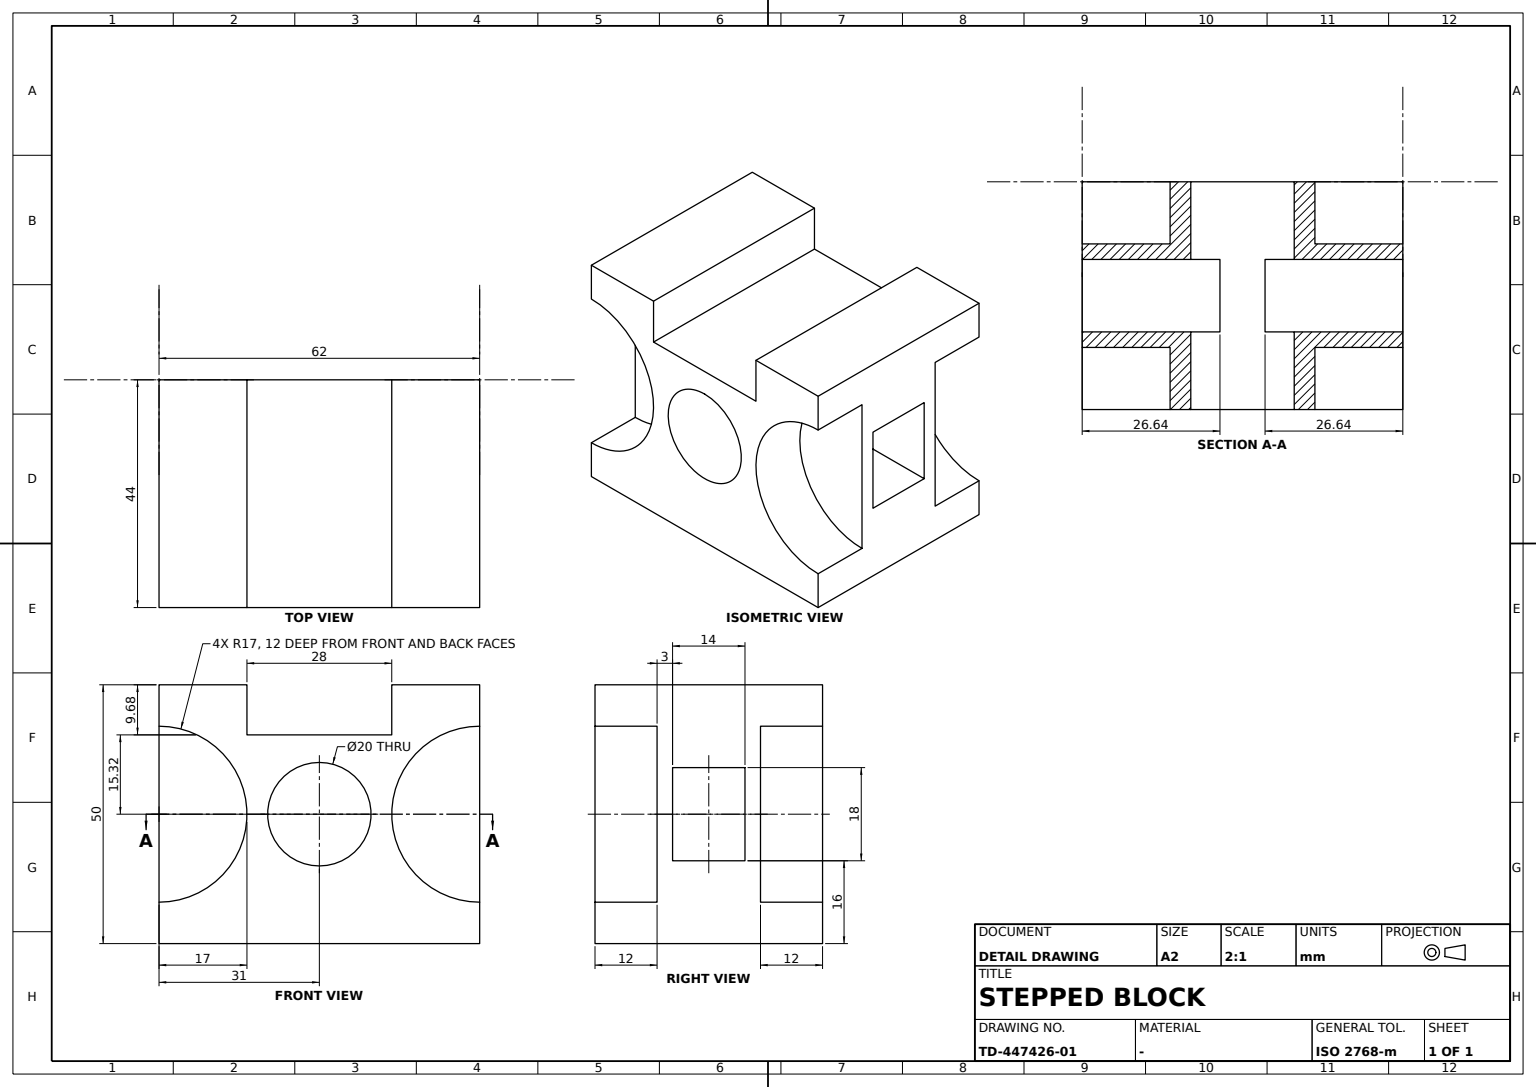
ISO-10303-21;
HEADER;
FILE_DESCRIPTION((''),'2;1');
FILE_NAME('','',(''),(''),'','','');
FILE_SCHEMA(('AUTOMOTIVE_DESIGN'));
ENDSEC;
DATA;
#1=APPLICATION_CONTEXT('');
#2=PRODUCT_CONTEXT('',#1,'mechanical');
#3=PRODUCT('','','',(#2));
#4=PRODUCT_DEFINITION_FORMATION('','',#3);
#5=PRODUCT_DEFINITION_CONTEXT('',#1,'design');
#6=PRODUCT_DEFINITION('','',#4,#5);
#7=PRODUCT_DEFINITION_SHAPE('','',#6);
#8=(LENGTH_UNIT()NAMED_UNIT(*)SI_UNIT(.MILLI.,.METRE.));
#9=(NAMED_UNIT(*)PLANE_ANGLE_UNIT()SI_UNIT($,.RADIAN.));
#10=(NAMED_UNIT(*)SI_UNIT($,.STERADIAN.)SOLID_ANGLE_UNIT());
#11=UNCERTAINTY_MEASURE_WITH_UNIT(LENGTH_MEASURE(0.005),#8,'distance_accuracy_value','');
#12=(GEOMETRIC_REPRESENTATION_CONTEXT(3)GLOBAL_UNCERTAINTY_ASSIGNED_CONTEXT((#11))GLOBAL_UNIT_ASSIGNED_CONTEXT((#8,#9,#10))REPRESENTATION_CONTEXT('',''));
#13=CARTESIAN_POINT('',(31.,-29.,-9.));
#14=VERTEX_POINT('',#13);
#15=CARTESIAN_POINT('',(31.,-29.,9.));
#16=VERTEX_POINT('',#15);
#17=DIRECTION('',(0.,0.,1.));
#18=VECTOR('',#17,1000.);
#19=LINE('',#13,#18);
#20=EDGE_CURVE('',#14,#16,#19,.T.);
#21=ORIENTED_EDGE('',*,*,#20,.F.);
#22=CARTESIAN_POINT('',(4.358899,-29.,-9.));
#23=VERTEX_POINT('',#22);
#24=DIRECTION('',(-1.,0.,0.));
#25=VECTOR('',#24,1000.);
#26=LINE('',#13,#25);
#27=EDGE_CURVE('',#14,#23,#26,.T.);
#28=ORIENTED_EDGE('',*,*,#27,.T.);
#29=CARTESIAN_POINT('',(4.358899,-29.,9.));
#30=VERTEX_POINT('',#29);
#31=CARTESIAN_POINT('',(0.,-29.,0.));
#32=DIRECTION('',(0.,-1.,0.));
#33=DIRECTION('',(0.,0.,-1.));
#34=AXIS2_PLACEMENT_3D('',#31,#32,#33);
#35=CIRCLE('',#34,10.);
#36=EDGE_CURVE('',#23,#30,#35,.T.);
#37=ORIENTED_EDGE('',*,*,#36,.T.);
#38=LINE('',#15,#25);
#39=EDGE_CURVE('',#16,#30,#38,.T.);
#40=ORIENTED_EDGE('',*,*,#39,.F.);
#41=EDGE_LOOP('',(#21,#28,#37,#40));
#42=FACE_BOUND('',#41,.T.);
#43=AXIS2_PLACEMENT_3D('',#13,#32,#17);
#44=PLANE('',#43);
#45=ADVANCED_FACE('',(#42),#44,.F.);
#46=CARTESIAN_POINT('',(14.,-44.,25.));
#47=VERTEX_POINT('',#46);
#48=CARTESIAN_POINT('',(14.,-44.,15.322407));
#49=VERTEX_POINT('',#48);
#50=VECTOR('',#33,1000.);
#51=LINE('',#46,#50);
#52=EDGE_CURVE('',#47,#49,#51,.T.);
#53=ORIENTED_EDGE('',*,*,#52,.F.);
#54=CARTESIAN_POINT('',(14.,0.,25.));
#55=VERTEX_POINT('',#54);
#56=VECTOR('',#32,1000.);
#57=LINE('',#54,#56);
#58=EDGE_CURVE('',#55,#47,#57,.T.);
#59=ORIENTED_EDGE('',*,*,#58,.F.);
#60=CARTESIAN_POINT('',(14.,0.,15.322407));
#61=VERTEX_POINT('',#60);
#62=LINE('',#54,#50);
#63=EDGE_CURVE('',#55,#61,#62,.T.);
#64=ORIENTED_EDGE('',*,*,#63,.T.);
#65=LINE('',#60,#56);
#66=EDGE_CURVE('',#61,#49,#65,.T.);
#67=ORIENTED_EDGE('',*,*,#66,.T.);
#68=EDGE_LOOP('',(#53,#59,#64,#67));
#69=FACE_BOUND('',#68,.T.);
#70=AXIS2_PLACEMENT_3D('',#54,#24,#33);
#71=PLANE('',#70);
#72=ADVANCED_FACE('',(#69),#71,.T.);
#73=CARTESIAN_POINT('',(-14.,0.,25.));
#74=VERTEX_POINT('',#73);
#75=CARTESIAN_POINT('',(-14.,-44.,25.));
#76=VERTEX_POINT('',#75);
#77=LINE('',#73,#56);
#78=EDGE_CURVE('',#74,#76,#77,.T.);
#79=ORIENTED_EDGE('',*,*,#78,.F.);
#80=CARTESIAN_POINT('',(-31.,0.,25.));
#81=VERTEX_POINT('',#80);
#82=LINE('',#73,#25);
#83=EDGE_CURVE('',#74,#81,#82,.T.);
#84=ORIENTED_EDGE('',*,*,#83,.T.);
#85=CARTESIAN_POINT('',(-31.,-44.,25.));
#86=VERTEX_POINT('',#85);
#87=LINE('',#80,#56);
#88=EDGE_CURVE('',#81,#86,#87,.T.);
#89=ORIENTED_EDGE('',*,*,#88,.T.);
#90=LINE('',#75,#25);
#91=EDGE_CURVE('',#76,#86,#90,.T.);
#92=ORIENTED_EDGE('',*,*,#91,.F.);
#93=EDGE_LOOP('',(#79,#84,#89,#92));
#94=FACE_BOUND('',#93,.T.);
#95=AXIS2_PLACEMENT_3D('',#73,#17,#24);
#96=PLANE('',#95);
#97=ADVANCED_FACE('',(#94),#96,.T.);
#98=CARTESIAN_POINT('',(0.,0.,10.));
#99=VERTEX_POINT('',#98);
#100=CARTESIAN_POINT('',(0.,0.,0.));
#101=DIRECTION('',(0.,1.,0.));
#102=AXIS2_PLACEMENT_3D('',#100,#101,#17);
#103=CIRCLE('',#102,10.);
#104=EDGE_CURVE('',#99,#99,#103,.T.);
#105=ORIENTED_EDGE('',*,*,#104,.F.);
#106=EDGE_LOOP('',(#105));
#107=FACE_BOUND('',#106,.T.);
#108=ORIENTED_EDGE('',*,*,#63,.F.);
#109=CARTESIAN_POINT('',(31.,0.,25.));
#110=VERTEX_POINT('',#109);
#111=EDGE_CURVE('',#110,#55,#82,.T.);
#112=ORIENTED_EDGE('',*,*,#111,.F.);
#113=CARTESIAN_POINT('',(31.,0.,17.));
#114=VERTEX_POINT('',#113);
#115=CARTESIAN_POINT('',(31.,0.,-25.));
#116=LINE('',#115,#18);
#117=EDGE_CURVE('',#114,#110,#116,.T.);
#118=ORIENTED_EDGE('',*,*,#117,.F.);
#119=CARTESIAN_POINT('',(31.,0.,-17.));
#120=VERTEX_POINT('',#119);
#121=CARTESIAN_POINT('',(31.,0.,0.));
#122=AXIS2_PLACEMENT_3D('',#121,#101,#17);
#123=CIRCLE('',#122,17.);
#124=EDGE_CURVE('',#120,#114,#123,.T.);
#125=ORIENTED_EDGE('',*,*,#124,.F.);
#126=VERTEX_POINT('',#115);
#127=EDGE_CURVE('',#126,#120,#116,.T.);
#128=ORIENTED_EDGE('',*,*,#127,.F.);
#129=CARTESIAN_POINT('',(-31.,0.,-25.));
#130=VERTEX_POINT('',#129);
#131=DIRECTION('',(1.,0.,0.));
#132=VECTOR('',#131,1000.);
#133=LINE('',#129,#132);
#134=EDGE_CURVE('',#130,#126,#133,.T.);
#135=ORIENTED_EDGE('',*,*,#134,.F.);
#136=CARTESIAN_POINT('',(-31.,0.,-17.));
#137=VERTEX_POINT('',#136);
#138=LINE('',#80,#50);
#139=EDGE_CURVE('',#137,#130,#138,.T.);
#140=ORIENTED_EDGE('',*,*,#139,.F.);
#141=CARTESIAN_POINT('',(-31.,0.,17.));
#142=VERTEX_POINT('',#141);
#143=CARTESIAN_POINT('',(-31.,0.,0.));
#144=AXIS2_PLACEMENT_3D('',#143,#101,#17);
#145=CIRCLE('',#144,17.);
#146=EDGE_CURVE('',#142,#137,#145,.T.);
#147=ORIENTED_EDGE('',*,*,#146,.F.);
#148=EDGE_CURVE('',#81,#142,#138,.T.);
#149=ORIENTED_EDGE('',*,*,#148,.F.);
#150=ORIENTED_EDGE('',*,*,#83,.F.);
#151=CARTESIAN_POINT('',(-14.,0.,15.322407));
#152=VERTEX_POINT('',#151);
#153=LINE('',#151,#18);
#154=EDGE_CURVE('',#152,#74,#153,.T.);
#155=ORIENTED_EDGE('',*,*,#154,.F.);
#156=LINE('',#60,#25);
#157=EDGE_CURVE('',#61,#152,#156,.T.);
#158=ORIENTED_EDGE('',*,*,#157,.F.);
#159=EDGE_LOOP('',(#108,#112,#118,#125,#128,#135,#140,#147,#149,#150,#155,#158));
#160=FACE_BOUND('',#159,.T.);
#161=AXIS2_PLACEMENT_3D('',#100,#101,#24);
#162=PLANE('',#161);
#163=ADVANCED_FACE('',(#107,#160),#162,.T.);
#164=CARTESIAN_POINT('',(-31.,-32.,-17.));
#165=VERTEX_POINT('',#164);
#166=CARTESIAN_POINT('',(-31.,-32.,17.));
#167=VERTEX_POINT('',#166);
#168=CARTESIAN_POINT('',(-31.,-32.,25.));
#169=LINE('',#168,#18);
#170=EDGE_CURVE('',#165,#167,#169,.T.);
#171=ORIENTED_EDGE('',*,*,#170,.F.);
#172=CARTESIAN_POINT('',(-31.,-32.,0.));
#173=AXIS2_PLACEMENT_3D('',#172,#32,#33);
#174=CIRCLE('',#173,17.);
#175=EDGE_CURVE('',#165,#167,#174,.T.);
#176=ORIENTED_EDGE('',*,*,#175,.T.);
#177=EDGE_LOOP('',(#171,#176));
#178=FACE_BOUND('',#177,.T.);
#179=CARTESIAN_POINT('',(0.,-32.,0.));
#180=AXIS2_PLACEMENT_3D('',#179,#32,#131);
#181=PLANE('',#180);
#182=ADVANCED_FACE('',(#178),#181,.T.);
#183=CARTESIAN_POINT('',(-31.,-44.,-25.));
#184=VERTEX_POINT('',#183);
#185=CARTESIAN_POINT('',(31.,-44.,-25.));
#186=VERTEX_POINT('',#185);
#187=LINE('',#183,#132);
#188=EDGE_CURVE('',#184,#186,#187,.T.);
#189=ORIENTED_EDGE('',*,*,#188,.F.);
#190=LINE('',#129,#56);
#191=EDGE_CURVE('',#130,#184,#190,.T.);
#192=ORIENTED_EDGE('',*,*,#191,.F.);
#193=ORIENTED_EDGE('',*,*,#134,.T.);
#194=LINE('',#115,#56);
#195=EDGE_CURVE('',#126,#186,#194,.T.);
#196=ORIENTED_EDGE('',*,*,#195,.T.);
#197=EDGE_LOOP('',(#189,#192,#193,#196));
#198=FACE_BOUND('',#197,.T.);
#199=AXIS2_PLACEMENT_3D('',#129,#33,#131);
#200=PLANE('',#199);
#201=ADVANCED_FACE('',(#198),#200,.T.);
#202=CARTESIAN_POINT('',(-31.,-15.,9.));
#203=VERTEX_POINT('',#202);
#204=CARTESIAN_POINT('',(-31.,-15.,-9.));
#205=VERTEX_POINT('',#204);
#206=CARTESIAN_POINT('',(-31.,-15.,25.));
#207=LINE('',#206,#50);
#208=EDGE_CURVE('',#203,#205,#207,.T.);
#209=ORIENTED_EDGE('',*,*,#208,.T.);
#210=CARTESIAN_POINT('',(-4.358899,-15.,-9.));
#211=VERTEX_POINT('',#210);
#212=CARTESIAN_POINT('',(31.,-15.,-9.));
#213=LINE('',#212,#25);
#214=EDGE_CURVE('',#211,#205,#213,.T.);
#215=ORIENTED_EDGE('',*,*,#214,.F.);
#216=CARTESIAN_POINT('',(-4.358899,-15.,9.));
#217=VERTEX_POINT('',#216);
#218=CARTESIAN_POINT('',(0.,-15.,0.));
#219=AXIS2_PLACEMENT_3D('',#218,#101,#17);
#220=CIRCLE('',#219,10.);
#221=EDGE_CURVE('',#211,#217,#220,.T.);
#222=ORIENTED_EDGE('',*,*,#221,.T.);
#223=CARTESIAN_POINT('',(31.,-15.,9.));
#224=LINE('',#223,#25);
#225=EDGE_CURVE('',#217,#203,#224,.T.);
#226=ORIENTED_EDGE('',*,*,#225,.T.);
#227=EDGE_LOOP('',(#209,#215,#222,#226));
#228=FACE_BOUND('',#227,.T.);
#229=AXIS2_PLACEMENT_3D('',#223,#101,#33);
#230=PLANE('',#229);
#231=ADVANCED_FACE('',(#228),#230,.F.);
#232=CARTESIAN_POINT('',(31.,-32.,17.));
#233=VERTEX_POINT('',#232);
#234=CARTESIAN_POINT('',(31.,-32.,-17.));
#235=VERTEX_POINT('',#234);
#236=CARTESIAN_POINT('',(31.,-32.,0.));
#237=AXIS2_PLACEMENT_3D('',#236,#32,#33);
#238=CIRCLE('',#237,17.);
#239=EDGE_CURVE('',#233,#235,#238,.T.);
#240=ORIENTED_EDGE('',*,*,#239,.F.);
#241=CARTESIAN_POINT('',(31.,-44.,17.));
#242=VERTEX_POINT('',#241);
#243=VECTOR('',#101,1000.);
#244=LINE('',#241,#243);
#245=EDGE_CURVE('',#233,#242,#244,.F.);
#246=ORIENTED_EDGE('',*,*,#245,.T.);
#247=CARTESIAN_POINT('',(31.,-44.,-17.));
#248=VERTEX_POINT('',#247);
#249=CARTESIAN_POINT('',(31.,-44.,0.));
#250=AXIS2_PLACEMENT_3D('',#249,#101,#17);
#251=CIRCLE('',#250,17.);
#252=EDGE_CURVE('',#242,#248,#251,.F.);
#253=ORIENTED_EDGE('',*,*,#252,.T.);
#254=LINE('',#247,#243);
#255=EDGE_CURVE('',#248,#235,#254,.T.);
#256=ORIENTED_EDGE('',*,*,#255,.T.);
#257=EDGE_LOOP('',(#240,#246,#253,#256));
#258=FACE_BOUND('',#257,.T.);
#259=CARTESIAN_POINT('',(31.,-6.,0.));
#260=AXIS2_PLACEMENT_3D('',#259,#101,#24);
#261=CYLINDRICAL_SURFACE('',#260,17.);
#262=ADVANCED_FACE('',(#258),#261,.F.);
#263=CARTESIAN_POINT('',(31.,-44.,25.));
#264=VERTEX_POINT('',#263);
#265=LINE('',#109,#56);
#266=EDGE_CURVE('',#110,#264,#265,.T.);
#267=ORIENTED_EDGE('',*,*,#266,.F.);
#268=ORIENTED_EDGE('',*,*,#111,.T.);
#269=ORIENTED_EDGE('',*,*,#58,.T.);
#270=EDGE_CURVE('',#264,#47,#90,.T.);
#271=ORIENTED_EDGE('',*,*,#270,.F.);
#272=EDGE_LOOP('',(#267,#268,#269,#271));
#273=FACE_BOUND('',#272,.T.);
#274=ADVANCED_FACE('',(#273),#96,.T.);
#275=ORIENTED_EDGE('',*,*,#175,.F.);
#276=CARTESIAN_POINT('',(-31.,-44.,-17.));
#277=VERTEX_POINT('',#276);
#278=LINE('',#276,#243);
#279=EDGE_CURVE('',#165,#277,#278,.F.);
#280=ORIENTED_EDGE('',*,*,#279,.T.);
#281=CARTESIAN_POINT('',(-31.,-44.,17.));
#282=VERTEX_POINT('',#281);
#283=CARTESIAN_POINT('',(-31.,-44.,0.));
#284=AXIS2_PLACEMENT_3D('',#283,#101,#17);
#285=CIRCLE('',#284,17.);
#286=EDGE_CURVE('',#277,#282,#285,.F.);
#287=ORIENTED_EDGE('',*,*,#286,.T.);
#288=LINE('',#281,#243);
#289=EDGE_CURVE('',#282,#167,#288,.T.);
#290=ORIENTED_EDGE('',*,*,#289,.T.);
#291=EDGE_LOOP('',(#275,#280,#287,#290));
#292=FACE_BOUND('',#291,.T.);
#293=CARTESIAN_POINT('',(-31.,-6.,0.));
#294=AXIS2_PLACEMENT_3D('',#293,#101,#24);
#295=CYLINDRICAL_SURFACE('',#294,17.);
#296=ADVANCED_FACE('',(#292),#295,.F.);
#297=VERTEX_POINT('',#223);
#298=CARTESIAN_POINT('',(4.358899,-15.,9.));
#299=VERTEX_POINT('',#298);
#300=EDGE_CURVE('',#297,#299,#224,.T.);
#301=ORIENTED_EDGE('',*,*,#300,.F.);
#302=LINE('',#15,#243);
#303=EDGE_CURVE('',#16,#297,#302,.T.);
#304=ORIENTED_EDGE('',*,*,#303,.F.);
#305=ORIENTED_EDGE('',*,*,#39,.T.);
#306=LINE('',#29,#56);
#307=EDGE_CURVE('',#299,#30,#306,.T.);
#308=ORIENTED_EDGE('',*,*,#307,.F.);
#309=EDGE_LOOP('',(#301,#304,#305,#308));
#310=FACE_BOUND('',#309,.T.);
#311=AXIS2_PLACEMENT_3D('',#15,#17,#101);
#312=PLANE('',#311);
#313=ADVANCED_FACE('',(#310),#312,.F.);
#314=CARTESIAN_POINT('',(-31.,-12.,17.));
#315=VERTEX_POINT('',#314);
#316=LINE('',#141,#243);
#317=EDGE_CURVE('',#142,#315,#316,.F.);
#318=ORIENTED_EDGE('',*,*,#317,.F.);
#319=ORIENTED_EDGE('',*,*,#146,.T.);
#320=CARTESIAN_POINT('',(-31.,-12.,-17.));
#321=VERTEX_POINT('',#320);
#322=LINE('',#136,#243);
#323=EDGE_CURVE('',#321,#137,#322,.T.);
#324=ORIENTED_EDGE('',*,*,#323,.F.);
#325=CARTESIAN_POINT('',(-31.,-12.,0.));
#326=AXIS2_PLACEMENT_3D('',#325,#101,#17);
#327=CIRCLE('',#326,17.);
#328=EDGE_CURVE('',#315,#321,#327,.T.);
#329=ORIENTED_EDGE('',*,*,#328,.F.);
#330=EDGE_LOOP('',(#318,#319,#324,#329));
#331=FACE_BOUND('',#330,.T.);
#332=ADVANCED_FACE('',(#331),#295,.F.);
#333=ORIENTED_EDGE('',*,*,#300,.T.);
#334=CARTESIAN_POINT('',(4.358899,-15.,-9.));
#335=VERTEX_POINT('',#334);
#336=EDGE_CURVE('',#299,#335,#220,.T.);
#337=ORIENTED_EDGE('',*,*,#336,.T.);
#338=VERTEX_POINT('',#212);
#339=EDGE_CURVE('',#338,#335,#213,.T.);
#340=ORIENTED_EDGE('',*,*,#339,.F.);
#341=LINE('',#223,#50);
#342=EDGE_CURVE('',#297,#338,#341,.T.);
#343=ORIENTED_EDGE('',*,*,#342,.F.);
#344=EDGE_LOOP('',(#333,#337,#340,#343));
#345=FACE_BOUND('',#344,.T.);
#346=ADVANCED_FACE('',(#345),#230,.F.);
#347=CARTESIAN_POINT('',(-31.,-29.,9.));
#348=VERTEX_POINT('',#347);
#349=CARTESIAN_POINT('',(-31.,0.,9.));
#350=LINE('',#349,#243);
#351=EDGE_CURVE('',#348,#203,#350,.T.);
#352=ORIENTED_EDGE('',*,*,#351,.F.);
#353=CARTESIAN_POINT('',(-31.,-29.,-9.));
#354=VERTEX_POINT('',#353);
#355=CARTESIAN_POINT('',(-31.,-29.,25.));
#356=LINE('',#355,#18);
#357=EDGE_CURVE('',#354,#348,#356,.T.);
#358=ORIENTED_EDGE('',*,*,#357,.F.);
#359=CARTESIAN_POINT('',(-31.,0.,-9.));
#360=LINE('',#359,#56);
#361=EDGE_CURVE('',#205,#354,#360,.T.);
#362=ORIENTED_EDGE('',*,*,#361,.F.);
#363=ORIENTED_EDGE('',*,*,#208,.F.);
#364=EDGE_LOOP('',(#352,#358,#362,#363));
#365=FACE_BOUND('',#364,.T.);
#366=LINE('',#85,#50);
#367=EDGE_CURVE('',#277,#184,#366,.T.);
#368=ORIENTED_EDGE('',*,*,#367,.F.);
#369=ORIENTED_EDGE('',*,*,#279,.F.);
#370=ORIENTED_EDGE('',*,*,#170,.T.);
#371=ORIENTED_EDGE('',*,*,#289,.F.);
#372=EDGE_CURVE('',#86,#282,#366,.T.);
#373=ORIENTED_EDGE('',*,*,#372,.F.);
#374=ORIENTED_EDGE('',*,*,#88,.F.);
#375=ORIENTED_EDGE('',*,*,#148,.T.);
#376=ORIENTED_EDGE('',*,*,#317,.T.);
#377=LINE('',#325,#18);
#378=EDGE_CURVE('',#321,#315,#377,.T.);
#379=ORIENTED_EDGE('',*,*,#378,.F.);
#380=ORIENTED_EDGE('',*,*,#323,.T.);
#381=ORIENTED_EDGE('',*,*,#139,.T.);
#382=ORIENTED_EDGE('',*,*,#191,.T.);
#383=EDGE_LOOP('',(#368,#369,#370,#371,#373,#374,#375,#376,#379,#380,#381,#382));
#384=FACE_BOUND('',#383,.T.);
#385=AXIS2_PLACEMENT_3D('',#80,#24,#33);
#386=PLANE('',#385);
#387=ADVANCED_FACE('',(#365,#384),#386,.T.);
#388=CARTESIAN_POINT('',(31.,-12.,17.));
#389=VERTEX_POINT('',#388);
#390=LINE('',#113,#243);
#391=EDGE_CURVE('',#114,#389,#390,.F.);
#392=ORIENTED_EDGE('',*,*,#391,.T.);
#393=CARTESIAN_POINT('',(31.,-12.,-17.));
#394=VERTEX_POINT('',#393);
#395=CARTESIAN_POINT('',(31.,-12.,0.));
#396=AXIS2_PLACEMENT_3D('',#395,#101,#17);
#397=CIRCLE('',#396,17.);
#398=EDGE_CURVE('',#394,#389,#397,.T.);
#399=ORIENTED_EDGE('',*,*,#398,.F.);
#400=LINE('',#119,#243);
#401=EDGE_CURVE('',#394,#120,#400,.T.);
#402=ORIENTED_EDGE('',*,*,#401,.T.);
#403=ORIENTED_EDGE('',*,*,#124,.T.);
#404=EDGE_LOOP('',(#392,#399,#402,#403));
#405=FACE_BOUND('',#404,.T.);
#406=ADVANCED_FACE('',(#405),#261,.F.);
#407=LINE('',#334,#56);
#408=EDGE_CURVE('',#335,#23,#407,.T.);
#409=ORIENTED_EDGE('',*,*,#408,.T.);
#410=ORIENTED_EDGE('',*,*,#27,.F.);
#411=LINE('',#212,#56);
#412=EDGE_CURVE('',#338,#14,#411,.T.);
#413=ORIENTED_EDGE('',*,*,#412,.F.);
#414=ORIENTED_EDGE('',*,*,#339,.T.);
#415=EDGE_LOOP('',(#409,#410,#413,#414));
#416=FACE_BOUND('',#415,.T.);
#417=AXIS2_PLACEMENT_3D('',#212,#33,#32);
#418=PLANE('',#417);
#419=ADVANCED_FACE('',(#416),#418,.F.);
#420=ORIENTED_EDGE('',*,*,#342,.T.);
#421=ORIENTED_EDGE('',*,*,#412,.T.);
#422=ORIENTED_EDGE('',*,*,#20,.T.);
#423=ORIENTED_EDGE('',*,*,#303,.T.);
#424=EDGE_LOOP('',(#420,#421,#422,#423));
#425=FACE_BOUND('',#424,.T.);
#426=LINE('',#185,#18);
#427=EDGE_CURVE('',#242,#264,#426,.T.);
#428=ORIENTED_EDGE('',*,*,#427,.F.);
#429=ORIENTED_EDGE('',*,*,#245,.F.);
#430=CARTESIAN_POINT('',(31.,-32.,-25.));
#431=LINE('',#430,#50);
#432=EDGE_CURVE('',#233,#235,#431,.T.);
#433=ORIENTED_EDGE('',*,*,#432,.T.);
#434=ORIENTED_EDGE('',*,*,#255,.F.);
#435=EDGE_CURVE('',#186,#248,#426,.T.);
#436=ORIENTED_EDGE('',*,*,#435,.F.);
#437=ORIENTED_EDGE('',*,*,#195,.F.);
#438=ORIENTED_EDGE('',*,*,#127,.T.);
#439=ORIENTED_EDGE('',*,*,#401,.F.);
#440=LINE('',#395,#50);
#441=EDGE_CURVE('',#389,#394,#440,.T.);
#442=ORIENTED_EDGE('',*,*,#441,.F.);
#443=ORIENTED_EDGE('',*,*,#391,.F.);
#444=ORIENTED_EDGE('',*,*,#117,.T.);
#445=ORIENTED_EDGE('',*,*,#266,.T.);
#446=EDGE_LOOP('',(#428,#429,#433,#434,#436,#437,#438,#439,#442,#443,#444,#445));
#447=FACE_BOUND('',#446,.T.);
#448=AXIS2_PLACEMENT_3D('',#115,#131,#17);
#449=PLANE('',#448);
#450=ADVANCED_FACE('',(#425,#447),#449,.T.);
#451=CARTESIAN_POINT('',(0.,-44.,10.));
#452=VERTEX_POINT('',#451);
#453=CARTESIAN_POINT('',(0.,-44.,0.));
#454=AXIS2_PLACEMENT_3D('',#453,#101,#17);
#455=CIRCLE('',#454,10.);
#456=EDGE_CURVE('',#452,#452,#455,.F.);
#457=ORIENTED_EDGE('',*,*,#456,.F.);
#458=EDGE_LOOP('',(#457));
#459=FACE_BOUND('',#458,.T.);
#460=ORIENTED_EDGE('',*,*,#435,.T.);
#461=ORIENTED_EDGE('',*,*,#252,.F.);
#462=ORIENTED_EDGE('',*,*,#427,.T.);
#463=ORIENTED_EDGE('',*,*,#270,.T.);
#464=ORIENTED_EDGE('',*,*,#52,.T.);
#465=CARTESIAN_POINT('',(-14.,-44.,15.322407));
#466=VERTEX_POINT('',#465);
#467=LINE('',#48,#25);
#468=EDGE_CURVE('',#49,#466,#467,.T.);
#469=ORIENTED_EDGE('',*,*,#468,.T.);
#470=LINE('',#465,#18);
#471=EDGE_CURVE('',#466,#76,#470,.T.);
#472=ORIENTED_EDGE('',*,*,#471,.T.);
#473=ORIENTED_EDGE('',*,*,#91,.T.);
#474=ORIENTED_EDGE('',*,*,#372,.T.);
#475=ORIENTED_EDGE('',*,*,#286,.F.);
#476=ORIENTED_EDGE('',*,*,#367,.T.);
#477=ORIENTED_EDGE('',*,*,#188,.T.);
#478=EDGE_LOOP('',(#460,#461,#462,#463,#464,#469,#472,#473,#474,#475,#476,#477));
#479=FACE_BOUND('',#478,.T.);
#480=AXIS2_PLACEMENT_3D('',#453,#101,#24);
#481=PLANE('',#480);
#482=ADVANCED_FACE('',(#459,#479),#481,.F.);
#483=ORIENTED_EDGE('',*,*,#398,.T.);
#484=ORIENTED_EDGE('',*,*,#441,.T.);
#485=EDGE_LOOP('',(#483,#484));
#486=FACE_BOUND('',#485,.T.);
#487=CARTESIAN_POINT('',(0.,-12.,0.));
#488=AXIS2_PLACEMENT_3D('',#487,#101,#24);
#489=PLANE('',#488);
#490=ADVANCED_FACE('',(#486),#489,.T.);
#491=ORIENTED_EDGE('',*,*,#351,.T.);
#492=ORIENTED_EDGE('',*,*,#225,.F.);
#493=CARTESIAN_POINT('',(-4.358899,-29.,9.));
#494=VERTEX_POINT('',#493);
#495=LINE('',#493,#56);
#496=EDGE_CURVE('',#494,#217,#495,.F.);
#497=ORIENTED_EDGE('',*,*,#496,.F.);
#498=EDGE_CURVE('',#494,#348,#38,.T.);
#499=ORIENTED_EDGE('',*,*,#498,.T.);
#500=EDGE_LOOP('',(#491,#492,#497,#499));
#501=FACE_BOUND('',#500,.T.);
#502=ADVANCED_FACE('',(#501),#312,.F.);
#503=CARTESIAN_POINT('',(-4.358899,-29.,-9.));
#504=VERTEX_POINT('',#503);
#505=EDGE_CURVE('',#494,#504,#35,.T.);
#506=ORIENTED_EDGE('',*,*,#505,.T.);
#507=EDGE_CURVE('',#504,#354,#26,.T.);
#508=ORIENTED_EDGE('',*,*,#507,.T.);
#509=ORIENTED_EDGE('',*,*,#357,.T.);
#510=ORIENTED_EDGE('',*,*,#498,.F.);
#511=EDGE_LOOP('',(#506,#508,#509,#510));
#512=FACE_BOUND('',#511,.T.);
#513=ADVANCED_FACE('',(#512),#44,.F.);
#514=ORIENTED_EDGE('',*,*,#468,.F.);
#515=ORIENTED_EDGE('',*,*,#66,.F.);
#516=ORIENTED_EDGE('',*,*,#157,.T.);
#517=LINE('',#151,#56);
#518=EDGE_CURVE('',#152,#466,#517,.T.);
#519=ORIENTED_EDGE('',*,*,#518,.T.);
#520=EDGE_LOOP('',(#514,#515,#516,#519));
#521=FACE_BOUND('',#520,.T.);
#522=AXIS2_PLACEMENT_3D('',#60,#17,#24);
#523=PLANE('',#522);
#524=ADVANCED_FACE('',(#521),#523,.T.);
#525=ORIENTED_EDGE('',*,*,#214,.T.);
#526=ORIENTED_EDGE('',*,*,#361,.T.);
#527=ORIENTED_EDGE('',*,*,#507,.F.);
#528=LINE('',#210,#56);
#529=EDGE_CURVE('',#504,#211,#528,.F.);
#530=ORIENTED_EDGE('',*,*,#529,.T.);
#531=EDGE_LOOP('',(#525,#526,#527,#530));
#532=FACE_BOUND('',#531,.T.);
#533=ADVANCED_FACE('',(#532),#418,.F.);
#534=ORIENTED_EDGE('',*,*,#328,.T.);
#535=ORIENTED_EDGE('',*,*,#378,.T.);
#536=EDGE_LOOP('',(#534,#535));
#537=FACE_BOUND('',#536,.T.);
#538=ADVANCED_FACE('',(#537),#489,.T.);
#539=ORIENTED_EDGE('',*,*,#78,.T.);
#540=ORIENTED_EDGE('',*,*,#471,.F.);
#541=ORIENTED_EDGE('',*,*,#518,.F.);
#542=ORIENTED_EDGE('',*,*,#154,.T.);
#543=EDGE_LOOP('',(#539,#540,#541,#542));
#544=FACE_BOUND('',#543,.T.);
#545=AXIS2_PLACEMENT_3D('',#151,#131,#17);
#546=PLANE('',#545);
#547=ADVANCED_FACE('',(#544),#546,.T.);
#548=ORIENTED_EDGE('',*,*,#36,.F.);
#549=ORIENTED_EDGE('',*,*,#408,.F.);
#550=ORIENTED_EDGE('',*,*,#336,.F.);
#551=ORIENTED_EDGE('',*,*,#307,.T.);
#552=EDGE_LOOP('',(#548,#549,#550,#551));
#553=FACE_BOUND('',#552,.T.);
#554=ORIENTED_EDGE('',*,*,#221,.F.);
#555=ORIENTED_EDGE('',*,*,#529,.F.);
#556=ORIENTED_EDGE('',*,*,#505,.F.);
#557=ORIENTED_EDGE('',*,*,#496,.T.);
#558=EDGE_LOOP('',(#554,#555,#556,#557));
#559=FACE_BOUND('',#558,.T.);
#560=ORIENTED_EDGE('',*,*,#456,.T.);
#561=EDGE_LOOP('',(#560));
#562=FACE_BOUND('',#561,.T.);
#563=ORIENTED_EDGE('',*,*,#104,.T.);
#564=EDGE_LOOP('',(#563));
#565=FACE_BOUND('',#564,.T.);
#566=CARTESIAN_POINT('',(0.,-21.34,0.));
#567=AXIS2_PLACEMENT_3D('',#566,#32,#131);
#568=CYLINDRICAL_SURFACE('',#567,10.);
#569=ADVANCED_FACE('',(#553,#559,#562,#565),#568,.F.);
#570=ORIENTED_EDGE('',*,*,#432,.F.);
#571=ORIENTED_EDGE('',*,*,#239,.T.);
#572=EDGE_LOOP('',(#570,#571));
#573=FACE_BOUND('',#572,.T.);
#574=ADVANCED_FACE('',(#573),#181,.T.);
#575=CLOSED_SHELL('',(#45,#72,#97,#163,#182,#201,#231,#262,#274,#296,#313,#332,#346,#387,#406,#419,#450,#482,#490,#502,#513,#524,#533,#538,#547,#569,#574));
#576=MANIFOLD_SOLID_BREP('',#575);
#577=ADVANCED_BREP_SHAPE_REPRESENTATION('',(#576),#12);
#578=SHAPE_DEFINITION_REPRESENTATION(#7,#577);
ENDSEC;
END-ISO-10303-21;
